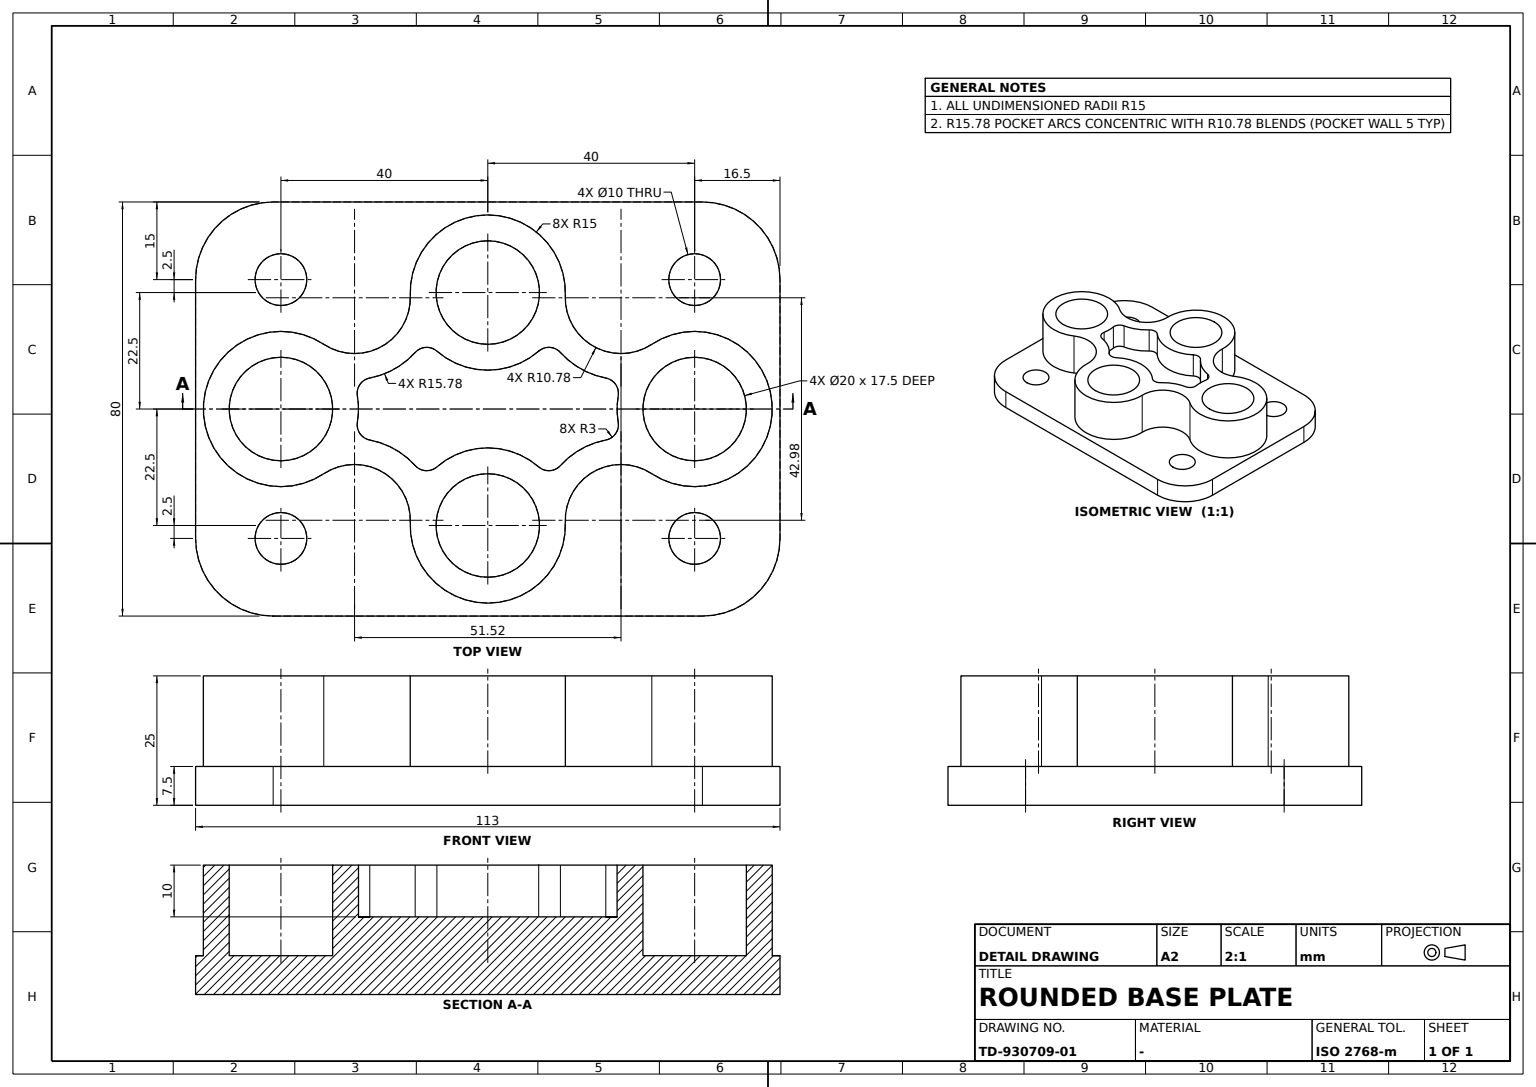
solid
v1 (-30,-40,7.5)
v2 (-30,-40,0)
e1 v1 v2 LINE
v3 (-20,-40,7.5)
e2 v1 v3 CIRCLE(AX(P(-25,-40,7.5),D(0,0,1),D(1,0,0)),5)
v4 (-20,-40,0)
e3 v3 v4 LINE
e4 v2 v4 CIRCLE(AX(P(-25,-40,0),D(0,0,1),D(1,0,0)),5)
face CYL(AX(P(-25,-40,3.75),D(0,0,-1),D(1,0,0)),5) rev [-e1 e2 e3 -e4]
v5 (-25,-56.5,0)
v6 (25,-56.5,0)
e5 v5 v6 LINE
v7 (-40,-41.5,0)
e6 v7 v5 CIRCLE(AX(P(-25,-41.5,0),D(0,0,1),D(1,0,0)),15)
v8 (-40,41.5,0)
e7 v8 v7 LINE
v9 (-25,56.5,0)
e8 v9 v8 CIRCLE(AX(P(-25,41.5,0),D(0,0,1),D(1,0,0)),15)
v10 (25,56.5,0)
e9 v10 v9 LINE
v11 (40,41.5,0)
e10 v11 v10 CIRCLE(AX(P(25,41.5,0),D(0,0,1),D(1,0,0)),15)
v12 (40,-41.5,0)
e11 v12 v11 LINE
e12 v6 v12 CIRCLE(AX(P(25,-41.5,0),D(0,0,1),D(1,0,0)),15)
e13 v4 v2 CIRCLE(AX(P(-25,-40,0),D(0,0,1),D(1,0,0)),5)
v13 (20,40,0)
v14 (30,40,0)
e14 v13 v14 CIRCLE(AX(P(25,40,0),D(0,0,1),D(1,0,0)),5)
e15 v14 v13 CIRCLE(AX(P(25,40,0),D(0,0,1),D(1,0,0)),5)
v15 (-30,40,0)
v16 (-20,40,0)
e16 v15 v16 CIRCLE(AX(P(-25,40,0),D(0,0,1),D(1,0,0)),5)
e17 v16 v15 CIRCLE(AX(P(-25,40,0),D(0,0,1),D(1,0,0)),5)
v17 (20,-40,0)
v18 (30,-40,0)
e18 v17 v18 CIRCLE(AX(P(25,-40,0),D(0,0,1),D(1,0,0)),5)
e19 v18 v17 CIRCLE(AX(P(25,-40,0),D(0,0,1),D(1,0,0)),5)
face PLANE(AX(P(0,0,0),D(0,0,1),D(1,0,0))) rev [-e5 -e6 -e7 -e8 -e9 -e10 -e11 -e12] [e13 e4] [e14 e15] [e16 e17] [e18 e19]
v19 (-25,56.5,7.5)
e20 v9 v19 LINE
v20 (-40,41.5,7.5)
e21 v8 v20 LINE
e22 v19 v20 CIRCLE(AX(P(-25,41.5,7.5),D(0,0,1),D(1,0,0)),15)
face CYL(AX(P(-25,41.5,3.75),D(0,0,-1),D(1,0,0)),15) [-e20 e8 e21 -e22]
v21 (-2.533656,25.215529,25)
v22 (-5.987763,22.81808,25)
e23 v21 v22 CIRCLE(AX(P(-3.040388,22.258635,25),D(0,0,1),D(1,0,0)),3)
v23 (-5.987763,22.81808,15)
e24 v22 v23 LINE
v24 (-2.533656,25.215529,15)
e25 v24 v23 CIRCLE(AX(P(-3.040388,22.258635,15),D(0,0,1),D(1,0,0)),3)
e26 v21 v24 LINE
face CYL(AX(P(-3.040388,22.258635,20),D(0,0,-1),D(1,0,0)),3) rev [e23 e24 -e25 -e26]
v25 (-11.180897,-9.842657,15)
v26 (-10.925713,-14.039501,15)
e27 v25 v26 CIRCLE(AX(P(-8.917076,-11.811189,15),D(0,0,1),D(1,0,0)),3)
v27 (-11.180897,-9.842657,25)
e28 v27 v25 LINE
v28 (-10.925713,-14.039501,25)
e29 v27 v28 CIRCLE(AX(P(-8.917076,-11.811189,25),D(0,0,1),D(1,0,0)),3)
e30 v28 v26 LINE
face CYL(AX(P(-8.917076,-11.811189,20),D(0,0,-1),D(1,0,0)),3) rev [-e27 -e28 e29 e30]
v29 (5.987763,-22.81808,15)
v30 (10.925713,-14.039501,15)
e31 v29 v30 CIRCLE(AX(P(21.49155,-25.760872,15),D(0,0,-1),D(1,0,0)),15.780603)
v31 (5.987763,-22.81808,25)
e32 v31 v29 LINE
v32 (10.925713,-14.039501,25)
e33 v31 v32 CIRCLE(AX(P(21.49155,-25.760872,25),D(0,0,-1),D(1,0,0)),15.780603)
e34 v32 v30 LINE
face CYL(AX(P(21.49155,-25.760872,20),D(0,0,-1),D(1,0,0)),15.780603) [-e31 -e32 e33 e34]
e35 v3 v1 CIRCLE(AX(P(-25,-40,7.5),D(0,0,1),D(1,0,0)),5)
face CYL(AX(P(-25,-40,3.75),D(0,0,-1),D(1,0,0)),5) rev [e35 e1 -e13 -e3]
v33 (-10,40,25)
v34 (10,40,25)
e36 v33 v34 CIRCLE(AX(P(0,40,25),D(0,0,1),D(1,0,0)),10)
v35 (10,40,7.5)
e37 v34 v35 LINE
v36 (-10,40,7.5)
e38 v36 v35 CIRCLE(AX(P(0,40,7.5),D(0,0,1),D(1,0,0)),10)
e39 v33 v36 LINE
face CYL(AX(P(0,40,16.25),D(0,0,-1),D(1,0,0)),10) rev [e36 e37 -e38 -e39]
v37 (15,-40,25)
v38 (12.504488,-31.715208,25)
e40 v37 v38 CIRCLE(AX(P(0,-40,25),D(0,0,1),D(1,0,0)),15)
v39 (15,-40,7.5)
e41 v37 v39 LINE
v40 (12.504488,-31.715208,7.5)
e42 v39 v40 CIRCLE(AX(P(0,-40,7.5),D(0,0,1),D(1,0,0)),15)
e43 v40 v38 LINE
face CYL(AX(P(0,-40,16.25),D(0,0,-1),D(1,0,0)),15) [-e40 e41 e42 e43]
e44 v35 v36 CIRCLE(AX(P(0,40,7.5),D(0,0,1),D(1,0,0)),10)
face PLANE(AX(P(0,0,7.5),D(0,0,1),D(1,0,0))) [e38 e44]
v41 (-12.5,0,25)
v42 (-12.5,0,7.5)
e45 v41 v42 LINE
v43 (-32.5,0,25)
e46 v41 v43 CIRCLE(AX(P(-22.5,0,25),D(0,0,1),D(1,0,0)),10)
v44 (-32.5,0,7.5)
e47 v43 v44 LINE
e48 v42 v44 CIRCLE(AX(P(-22.5,0,7.5),D(0,0,1),D(1,0,0)),10)
face CYL(AX(P(-22.5,0,16.25),D(0,0,-1),D(1,0,0)),10) rev [-e45 e46 e47 -e48]
e49 v34 v33 CIRCLE(AX(P(0,40,25),D(0,0,1),D(1,0,0)),10)
face CYL(AX(P(0,40,16.25),D(0,0,-1),D(1,0,0)),10) rev [-e44 -e37 e49 e39]
v45 (11.180897,-9.842657,25)
v46 (11.180897,9.842657,25)
e50 v45 v46 CIRCLE(AX(P(22.5,0,25),D(0,0,-1),D(1,0,0)),15)
v47 (11.180897,9.842657,15)
e51 v46 v47 LINE
v48 (11.180897,-9.842657,15)
e52 v48 v47 CIRCLE(AX(P(22.5,0,15),D(0,0,-1),D(1,0,0)),15)
e53 v45 v48 LINE
face CYL(AX(P(22.5,0,20),D(0,0,-1),D(1,0,0)),15) [e50 e51 -e52 -e53]
v49 (-2.533656,-25.215529,15)
v50 (2.533656,-25.215529,15)
e54 v49 v50 CIRCLE(AX(P(0,-40,15),D(0,0,-1),D(1,0,0)),15)
e55 v50 v29 CIRCLE(AX(P(3.040388,-22.258635,15),D(0,0,1),D(1,0,0)),3)
v51 (11.917076,-11.811189,15)
e56 v30 v51 CIRCLE(AX(P(8.917076,-11.811189,15),D(0,0,1),D(1,0,0)),3)
e57 v51 v48 CIRCLE(AX(P(8.917076,-11.811189,15),D(0,0,1),D(1,0,0)),3)
v52 (11.917076,11.811189,15)
e58 v47 v52 CIRCLE(AX(P(8.917076,11.811189,15),D(0,0,1),D(1,0,0)),3)
v53 (10.925713,14.039501,15)
e59 v52 v53 CIRCLE(AX(P(8.917076,11.811189,15),D(0,0,1),D(1,0,0)),3)
v54 (5.987763,22.81808,15)
e60 v53 v54 CIRCLE(AX(P(21.49155,25.760872,15),D(0,0,-1),D(1,0,0)),15.780603)
v55 (2.533656,25.215529,15)
e61 v54 v55 CIRCLE(AX(P(3.040388,22.258635,15),D(0,0,1),D(1,0,0)),3)
e62 v55 v24 CIRCLE(AX(P(0,40,15),D(0,0,-1),D(1,0,0)),15)
v56 (-10.925713,14.039501,15)
e63 v23 v56 CIRCLE(AX(P(-21.49155,25.760872,15),D(0,0,-1),D(1,0,0)),15.780603)
v57 (-11.180897,9.842657,15)
e64 v56 v57 CIRCLE(AX(P(-8.917076,11.811189,15),D(0,0,1),D(1,0,0)),3)
v58 (-7.5,0,15)
e65 v57 v58 CIRCLE(AX(P(-22.5,0,15),D(0,0,-1),D(1,0,0)),15)
e66 v58 v25 CIRCLE(AX(P(-22.5,0,15),D(0,0,-1),D(1,0,0)),15)
v59 (-5.987763,-22.81808,15)
e67 v26 v59 CIRCLE(AX(P(-21.49155,-25.760872,15),D(0,0,-1),D(1,0,0)),15.780603)
e68 v59 v49 CIRCLE(AX(P(-3.040388,-22.258635,15),D(0,0,1),D(1,0,0)),3)
face PLANE(AX(P(0,0,15),D(0,0,1),D(1,0,0))) [e54 e55 e31 e56 e57 e52 e58 e59 e60 e61 e62 e25 e63 e64 e65 e66 e27 e67 e68]
v60 (-10,-40,7.5)
v61 (10,-40,7.5)
e69 v60 v61 CIRCLE(AX(P(0,-40,7.5),D(0,0,1),D(1,0,0)),10)
v62 (-10,-40,25)
e70 v62 v60 LINE
v63 (10,-40,25)
e71 v62 v63 CIRCLE(AX(P(0,-40,25),D(0,0,1),D(1,0,0)),10)
e72 v63 v61 LINE
face CYL(AX(P(0,-40,16.25),D(0,0,-1),D(1,0,0)),10) rev [-e69 -e70 e71 e72]
v64 (-5.987763,-22.81808,25)
e73 v64 v59 LINE
v65 (-2.533656,-25.215529,25)
e74 v64 v65 CIRCLE(AX(P(-3.040388,-22.258635,25),D(0,0,1),D(1,0,0)),3)
e75 v65 v49 LINE
face CYL(AX(P(-3.040388,-22.258635,20),D(0,0,-1),D(1,0,0)),3) rev [-e68 -e73 e74 e75]
v66 (32.5,0,7.5)
v67 (12.5,0,7.5)
e76 v66 v67 CIRCLE(AX(P(22.5,0,7.5),D(0,0,1),D(1,0,0)),10)
e77 v67 v66 CIRCLE(AX(P(22.5,0,7.5),D(0,0,1),D(1,0,0)),10)
face PLANE(AX(P(0,0,7.5),D(0,0,1),D(1,0,0))) [e76 e77]
v68 (12.5,0,25)
v69 (32.5,0,25)
e78 v68 v69 CIRCLE(AX(P(22.5,0,25),D(0,0,1),D(1,0,0)),10)
e79 v69 v68 CIRCLE(AX(P(22.5,0,25),D(0,0,1),D(1,0,0)),10)
e80 v63 v62 CIRCLE(AX(P(0,-40,25),D(0,0,1),D(1,0,0)),10)
e81 v43 v41 CIRCLE(AX(P(-22.5,0,25),D(0,0,1),D(1,0,0)),10)
v70 (37.5,0,25)
v71 (21.913251,14.98852,25)
e82 v70 v71 CIRCLE(AX(P(22.5,0,25),D(0,0,1),D(1,0,0)),15)
v72 (12.504488,31.715208,25)
e83 v71 v72 CIRCLE(AX(P(21.49155,25.760872,25),D(0,0,-1),D(1,0,0)),10.780603)
v73 (15,40,25)
e84 v72 v73 CIRCLE(AX(P(0,40,25),D(0,0,1),D(1,0,0)),15)
v74 (-15,40,25)
e85 v73 v74 CIRCLE(AX(P(0,40,25),D(0,0,1),D(1,0,0)),15)
v75 (-12.504488,31.715208,25)
e86 v74 v75 CIRCLE(AX(P(0,40,25),D(0,0,1),D(1,0,0)),15)
v76 (-10.710947,25.760872,25)
e87 v75 v76 CIRCLE(AX(P(-21.49155,25.760872,25),D(0,0,-1),D(1,0,0)),10.780603)
v77 (-21.913251,14.98852,25)
e88 v76 v77 CIRCLE(AX(P(-21.49155,25.760872,25),D(0,0,-1),D(1,0,0)),10.780603)
v78 (-21.913251,-14.98852,25)
e89 v77 v78 CIRCLE(AX(P(-22.5,0,25),D(0,0,1),D(1,0,0)),15)
v79 (-10.710947,-25.760872,25)
e90 v78 v79 CIRCLE(AX(P(-21.49155,-25.760872,25),D(0,0,-1),D(1,0,0)),10.780603)
v80 (-12.504488,-31.715208,25)
e91 v79 v80 CIRCLE(AX(P(-21.49155,-25.760872,25),D(0,0,-1),D(1,0,0)),10.780603)
v81 (-15,-40,25)
e92 v80 v81 CIRCLE(AX(P(0,-40,25),D(0,0,1),D(1,0,0)),15)
e93 v81 v37 CIRCLE(AX(P(0,-40,25),D(0,0,1),D(1,0,0)),15)
v82 (21.913251,-14.98852,25)
e94 v38 v82 CIRCLE(AX(P(21.49155,-25.760872,25),D(0,0,-1),D(1,0,0)),10.780603)
e95 v82 v70 CIRCLE(AX(P(22.5,0,25),D(0,0,1),D(1,0,0)),15)
v83 (-11.180897,9.842657,25)
v84 (-7.5,0,25)
e96 v83 v84 CIRCLE(AX(P(-22.5,0,25),D(0,0,-1),D(1,0,0)),15)
v85 (-10.925713,14.039501,25)
e97 v85 v83 CIRCLE(AX(P(-8.917076,11.811189,25),D(0,0,1),D(1,0,0)),3)
e98 v22 v85 CIRCLE(AX(P(-21.49155,25.760872,25),D(0,0,-1),D(1,0,0)),15.780603)
v86 (2.533656,25.215529,25)
e99 v86 v21 CIRCLE(AX(P(0,40,25),D(0,0,-1),D(1,0,0)),15)
v87 (5.987763,22.81808,25)
e100 v87 v86 CIRCLE(AX(P(3.040388,22.258635,25),D(0,0,1),D(1,0,0)),3)
v88 (10.925713,14.039501,25)
e101 v88 v87 CIRCLE(AX(P(21.49155,25.760872,25),D(0,0,-1),D(1,0,0)),15.780603)
v89 (11.917076,11.811189,25)
e102 v89 v88 CIRCLE(AX(P(8.917076,11.811189,25),D(0,0,1),D(1,0,0)),3)
e103 v46 v89 CIRCLE(AX(P(8.917076,11.811189,25),D(0,0,1),D(1,0,0)),3)
v90 (11.917076,-11.811189,25)
e104 v90 v45 CIRCLE(AX(P(8.917076,-11.811189,25),D(0,0,1),D(1,0,0)),3)
e105 v32 v90 CIRCLE(AX(P(8.917076,-11.811189,25),D(0,0,1),D(1,0,0)),3)
v91 (2.533656,-25.215529,25)
e106 v91 v31 CIRCLE(AX(P(3.040388,-22.258635,25),D(0,0,1),D(1,0,0)),3)
e107 v65 v91 CIRCLE(AX(P(0,-40,25),D(0,0,-1),D(1,0,0)),15)
e108 v28 v64 CIRCLE(AX(P(-21.49155,-25.760872,25),D(0,0,-1),D(1,0,0)),15.780603)
e109 v84 v27 CIRCLE(AX(P(-22.5,0,25),D(0,0,-1),D(1,0,0)),15)
face PLANE(AX(P(0,0,25),D(0,0,1),D(1,0,0))) [-e78 -e79] [-e71 -e80] [-e81 -e46] [-e36 -e49] [e82 e83 e84 e85 e86 e87 e88 e89 e90 e91 e92 e93 e40 e94 e95] [-e96 -e97 -e98 -e23 -e99 -e100 -e101 -e102 -e103 -e50 -e104 -e105 -e33 -e106 -e107 -e74 -e108 -e29 -e109]
e110 v87 v54 LINE
e111 v88 v53 LINE
face CYL(AX(P(21.49155,25.760872,20),D(0,0,-1),D(1,0,0)),15.780603) [e110 -e60 -e111 e101]
v92 (-10.710947,25.760872,7.5)
e112 v76 v92 LINE
v93 (-21.913251,14.98852,7.5)
e113 v92 v93 CIRCLE(AX(P(-21.49155,25.760872,7.5),D(0,0,-1),D(1,0,0)),10.780603)
e114 v93 v77 LINE
face CYL(AX(P(-21.49155,25.760872,16.25),D(0,0,-1),D(1,0,0)),10.780603) rev [-e88 e112 e113 e114]
v94 (21.913251,14.98852,7.5)
e115 v94 v71 LINE
v95 (37.5,0,7.5)
e116 v70 v95 LINE
e117 v95 v94 CIRCLE(AX(P(22.5,0,7.5),D(0,0,1),D(1,0,0)),15)
face CYL(AX(P(22.5,0,16.25),D(0,0,-1),D(1,0,0)),15) [e115 -e82 e116 e117]
e118 v83 v57 LINE
e119 v84 v58 LINE
face CYL(AX(P(-22.5,0,20),D(0,0,-1),D(1,0,0)),15) [-e65 -e118 e96 e119]
e120 v69 v66 LINE
e121 v68 v67 LINE
face CYL(AX(P(22.5,0,16.25),D(0,0,-1),D(1,0,0)),10) rev [e120 -e77 -e121 e78]
face CYL(AX(P(-21.49155,-25.760872,20),D(0,0,-1),D(1,0,0)),15.780603) [-e67 -e30 e108 e73]
e122 v91 v50 LINE
face CYL(AX(P(3.040388,-22.258635,20),D(0,0,-1),D(1,0,0)),3) rev [e32 -e55 -e122 e106]
e123 v85 v56 LINE
face CYL(AX(P(-21.49155,25.760872,20),D(0,0,-1),D(1,0,0)),15.780603) [e98 e123 -e63 -e24]
e124 v44 v42 CIRCLE(AX(P(-22.5,0,7.5),D(0,0,1),D(1,0,0)),10)
face PLANE(AX(P(0,0,7.5),D(0,0,1),D(1,0,0))) [e48 e124]
v96 (20,40,7.5)
e125 v96 v13 LINE
v97 (30,40,7.5)
e126 v96 v97 CIRCLE(AX(P(25,40,7.5),D(0,0,1),D(1,0,0)),5)
e127 v97 v14 LINE
face CYL(AX(P(25,40,3.75),D(0,0,-1),D(1,0,0)),5) rev [-e125 e126 e127 -e14]
v98 (20,-40,7.5)
v99 (30,-40,7.5)
e128 v98 v99 CIRCLE(AX(P(25,-40,7.5),D(0,0,1),D(1,0,0)),5)
e129 v99 v18 LINE
e130 v98 v17 LINE
face CYL(AX(P(25,-40,3.75),D(0,0,-1),D(1,0,0)),5) rev [e128 e129 -e18 -e130]
v100 (-40,-41.5,7.5)
e131 v7 v100 LINE
e132 v20 v100 LINE
face PLANE(AX(P(-40,-41.5,0),D(1,0,0),D(0,1,0))) rev [e7 e131 -e132 -e21]
e133 v86 v55 LINE
face CYL(AX(P(3.040388,22.258635,20),D(0,0,-1),D(1,0,0)),3) rev [e133 -e61 -e110 e100]
e134 v97 v96 CIRCLE(AX(P(25,40,7.5),D(0,0,1),D(1,0,0)),5)
face CYL(AX(P(25,40,3.75),D(0,0,-1),D(1,0,0)),5) rev [e125 -e15 -e127 e134]
v101 (25,-56.5,7.5)
e135 v6 v101 LINE
v102 (40,-41.5,7.5)
e136 v12 v102 LINE
e137 v101 v102 CIRCLE(AX(P(25,-41.5,7.5),D(0,0,1),D(1,0,0)),15)
face CYL(AX(P(25,-41.5,3.75),D(0,0,-1),D(1,0,0)),15) [-e135 e12 e136 -e137]
face CYL(AX(P(22.5,0,16.25),D(0,0,-1),D(1,0,0)),10) rev [-e120 e79 e121 -e76]
v103 (-10.710947,-25.760872,7.5)
v104 (-12.504488,-31.715208,7.5)
e138 v103 v104 CIRCLE(AX(P(-21.49155,-25.760872,7.5),D(0,0,-1),D(1,0,0)),10.780603)
e139 v104 v80 LINE
e140 v79 v103 LINE
face CYL(AX(P(-21.49155,-25.760872,16.25),D(0,0,-1),D(1,0,0)),10.780603) rev [e138 e139 -e91 e140]
e141 v90 v51 LINE
face CYL(AX(P(8.917076,-11.811189,20),D(0,0,-1),D(1,0,0)),3) rev [e105 e141 -e56 -e34]
e142 v89 v52 LINE
face CYL(AX(P(8.917076,11.811189,20),D(0,0,-1),D(1,0,0)),3) rev [e111 -e59 -e142 e102]
e143 v99 v98 CIRCLE(AX(P(25,-40,7.5),D(0,0,1),D(1,0,0)),5)
face CYL(AX(P(25,-40,3.75),D(0,0,-1),D(1,0,0)),5) rev [-e129 e143 e130 -e19]
v105 (-25,-56.5,7.5)
e144 v105 v101 LINE
v106 (40,41.5,7.5)
e145 v102 v106 LINE
v107 (25,56.5,7.5)
e146 v106 v107 CIRCLE(AX(P(25,41.5,7.5),D(0,0,1),D(1,0,0)),15)
e147 v107 v19 LINE
e148 v100 v105 CIRCLE(AX(P(-25,-41.5,7.5),D(0,0,1),D(1,0,0)),15)
v108 (-30,40,7.5)
v109 (-20,40,7.5)
e149 v108 v109 CIRCLE(AX(P(-25,40,7.5),D(0,0,1),D(1,0,0)),5)
e150 v109 v108 CIRCLE(AX(P(-25,40,7.5),D(0,0,1),D(1,0,0)),5)
v110 (-12.504488,31.715208,7.5)
e151 v110 v92 CIRCLE(AX(P(-21.49155,25.760872,7.5),D(0,0,-1),D(1,0,0)),10.780603)
v111 (-15,40,7.5)
e152 v111 v110 CIRCLE(AX(P(0,40,7.5),D(0,0,1),D(1,0,0)),15)
v112 (15,40,7.5)
e153 v112 v111 CIRCLE(AX(P(0,40,7.5),D(0,0,1),D(1,0,0)),15)
v113 (12.504488,31.715208,7.5)
e154 v113 v112 CIRCLE(AX(P(0,40,7.5),D(0,0,1),D(1,0,0)),15)
e155 v94 v113 CIRCLE(AX(P(21.49155,25.760872,7.5),D(0,0,-1),D(1,0,0)),10.780603)
v114 (21.913251,-14.98852,7.5)
e156 v114 v95 CIRCLE(AX(P(22.5,0,7.5),D(0,0,1),D(1,0,0)),15)
e157 v40 v114 CIRCLE(AX(P(21.49155,-25.760872,7.5),D(0,0,-1),D(1,0,0)),10.780603)
v115 (-15,-40,7.5)
e158 v115 v39 CIRCLE(AX(P(0,-40,7.5),D(0,0,1),D(1,0,0)),15)
e159 v104 v115 CIRCLE(AX(P(0,-40,7.5),D(0,0,1),D(1,0,0)),15)
v116 (-21.913251,-14.98852,7.5)
e160 v116 v103 CIRCLE(AX(P(-21.49155,-25.760872,7.5),D(0,0,-1),D(1,0,0)),10.780603)
e161 v93 v116 CIRCLE(AX(P(-22.5,0,7.5),D(0,0,1),D(1,0,0)),15)
face PLANE(AX(P(0,0,7.5),D(0,0,1),D(1,0,0))) [-e126 -e134] [e144 e137 e145 e146 e147 e22 e132 e148] [-e35 -e2] [-e143 -e128] [-e149 -e150] [-e151 -e152 -e153 -e154 -e155 -e117 -e156 -e157 -e42 -e158 -e159 -e138 -e160 -e161 -e113]
e162 v114 v82 LINE
face CYL(AX(P(21.49155,-25.760872,16.25),D(0,0,-1),D(1,0,0)),10.780603) rev [-e43 e157 e162 -e94]
face CYL(AX(P(-22.5,0,20),D(0,0,-1),D(1,0,0)),15) [e109 e28 -e66 -e119]
e163 v5 v105 LINE
face CYL(AX(P(-25,-41.5,3.75),D(0,0,-1),D(1,0,0)),15) [-e131 e6 e163 -e148]
e164 v73 v112 LINE
e165 v74 v111 LINE
face CYL(AX(P(0,40,16.25),D(0,0,-1),D(1,0,0)),15) [e164 e153 -e165 -e85]
e166 v81 v115 LINE
face CYL(AX(P(0,-40,16.25),D(0,0,-1),D(1,0,0)),15) [-e41 -e93 e166 e158]
e167 v116 v78 LINE
face CYL(AX(P(-22.5,0,16.25),D(0,0,-1),D(1,0,0)),15) [e167 -e89 -e114 e161]
face PLANE(AX(P(25,-56.5,0),D(0,1,0),D(-1,0,0))) rev [-e144 -e163 e5 e135]
face CYL(AX(P(0,-40,16.25),D(0,0,-1),D(1,0,0)),15) [e159 -e166 -e92 -e139]
e168 v113 v72 LINE
face CYL(AX(P(21.49155,25.760872,16.25),D(0,0,-1),D(1,0,0)),10.780603) rev [-e83 -e115 e155 e168]
face CYL(AX(P(22.5,0,16.25),D(0,0,-1),D(1,0,0)),15) [e156 -e116 -e95 -e162]
face CYL(AX(P(0,-40,20),D(0,0,-1),D(1,0,0)),15) [-e54 -e75 e107 e122]
face CYL(AX(P(8.917076,11.811189,20),D(0,0,-1),D(1,0,0)),3) rev [e103 e142 -e58 -e51]
e169 v110 v75 LINE
face CYL(AX(P(0,40,16.25),D(0,0,-1),D(1,0,0)),15) [e165 e152 e169 -e86]
e170 v108 v15 LINE
e171 v109 v16 LINE
face CYL(AX(P(-25,40,3.75),D(0,0,-1),D(1,0,0)),5) rev [-e16 -e170 e149 e171]
face CYL(AX(P(-22.5,0,16.25),D(0,0,-1),D(1,0,0)),10) rev [-e47 e81 e45 -e124]
face CYL(AX(P(0,40,20),D(0,0,-1),D(1,0,0)),15) [e99 e26 -e62 -e133]
face CYL(AX(P(-8.917076,11.811189,20),D(0,0,-1),D(1,0,0)),3) rev [-e123 e97 e118 -e64]
face CYL(AX(P(-25,40,3.75),D(0,0,-1),D(1,0,0)),5) rev [e150 e170 -e17 -e171]
e172 v10 v107 LINE
e173 v11 v106 LINE
face CYL(AX(P(25,41.5,3.75),D(0,0,-1),D(1,0,0)),15) [e10 e172 -e146 -e173]
face PLANE(AX(P(40,41.5,0),D(-1,0,0),D(0,-1,0))) rev [-e145 -e136 e11 e173]
face PLANE(AX(P(-25,56.5,0),D(0,-1,0),D(1,0,0))) rev [e9 e20 -e147 -e172]
e174 v61 v60 CIRCLE(AX(P(0,-40,7.5),D(0,0,1),D(1,0,0)),10)
face PLANE(AX(P(0,0,7.5),D(0,0,1),D(1,0,0))) [e174 e69]
face CYL(AX(P(-21.49155,25.760872,16.25),D(0,0,-1),D(1,0,0)),10.780603) rev [-e169 e151 -e112 -e87]
face CYL(AX(P(0,40,16.25),D(0,0,-1),D(1,0,0)),15) [-e84 -e168 e154 -e164]
face CYL(AX(P(0,-40,16.25),D(0,0,-1),D(1,0,0)),10) rev [e70 -e174 -e72 e80]
face CYL(AX(P(8.917076,-11.811189,20),D(0,0,-1),D(1,0,0)),3) rev [-e141 e104 e53 -e57]
face CYL(AX(P(-21.49155,-25.760872,16.25),D(0,0,-1),D(1,0,0)),10.780603) rev [-e140 -e90 -e167 e160]
